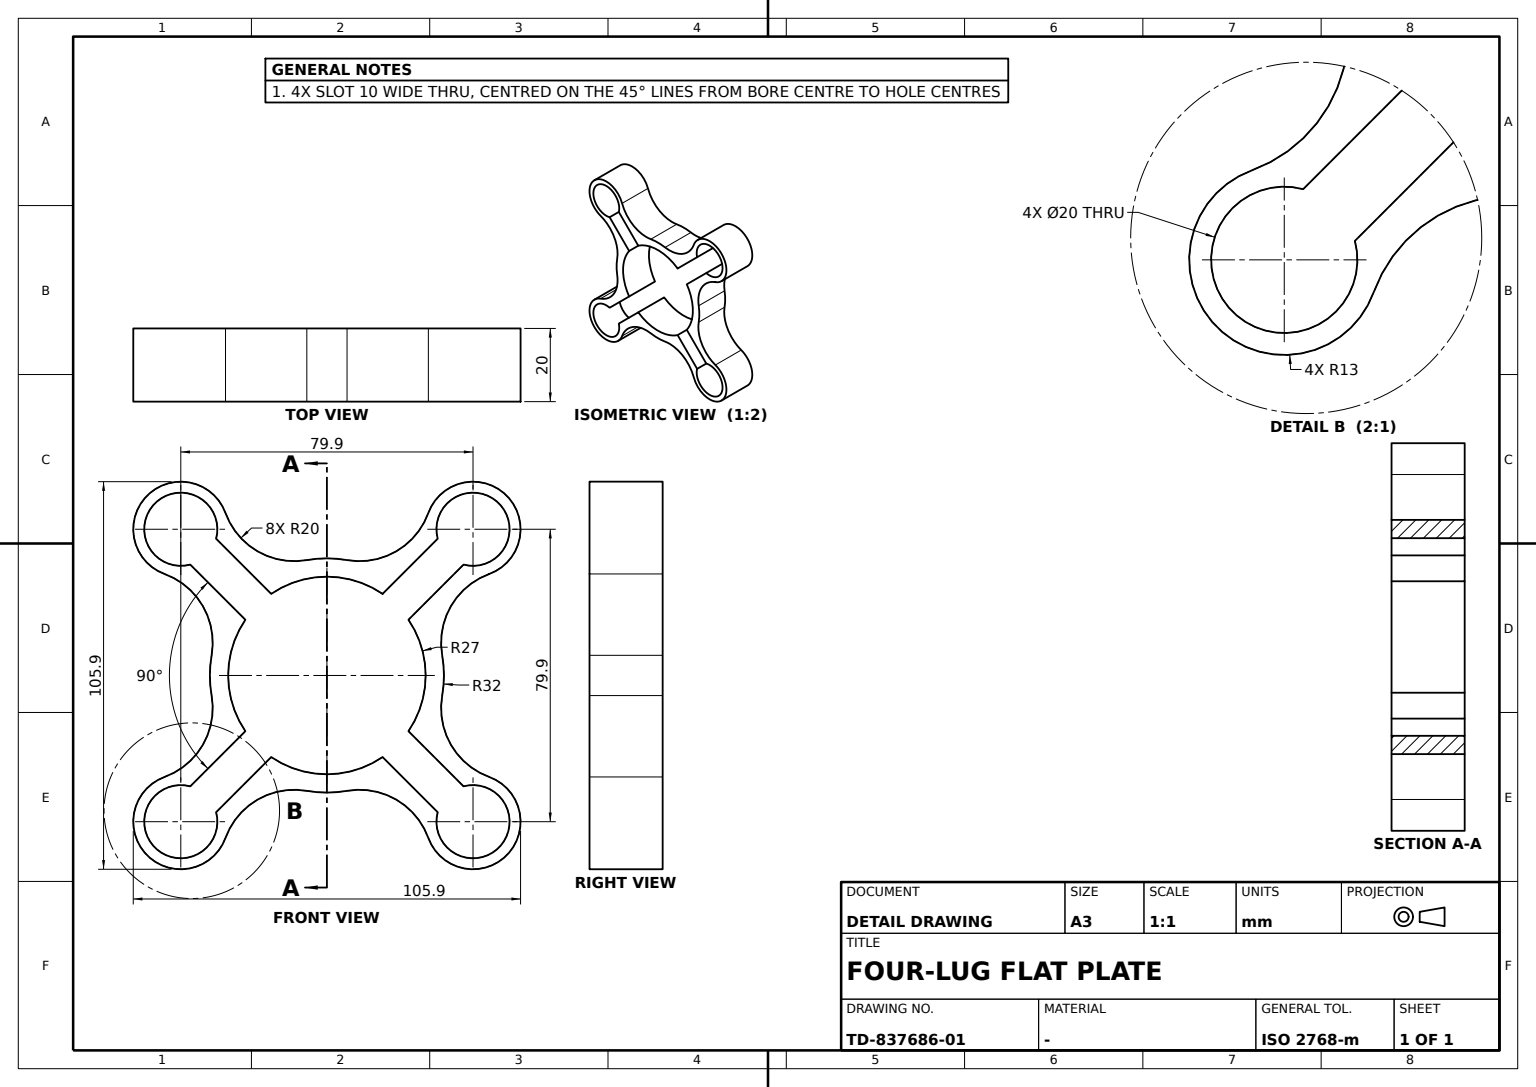
ISO-10303-21;
HEADER;
FILE_DESCRIPTION((''),'2;1');
FILE_NAME('','',(''),(''),'','','');
FILE_SCHEMA(('AUTOMOTIVE_DESIGN'));
ENDSEC;
DATA;
#1=APPLICATION_CONTEXT('');
#2=PRODUCT_CONTEXT('',#1,'mechanical');
#3=PRODUCT('','','',(#2));
#4=PRODUCT_DEFINITION_FORMATION('','',#3);
#5=PRODUCT_DEFINITION_CONTEXT('',#1,'design');
#6=PRODUCT_DEFINITION('','',#4,#5);
#7=PRODUCT_DEFINITION_SHAPE('','',#6);
#8=(LENGTH_UNIT()NAMED_UNIT(*)SI_UNIT(.MILLI.,.METRE.));
#9=(NAMED_UNIT(*)PLANE_ANGLE_UNIT()SI_UNIT($,.RADIAN.));
#10=(NAMED_UNIT(*)SI_UNIT($,.STERADIAN.)SOLID_ANGLE_UNIT());
#11=UNCERTAINTY_MEASURE_WITH_UNIT(LENGTH_MEASURE(0.005),#8,'distance_accuracy_value','');
#12=(GEOMETRIC_REPRESENTATION_CONTEXT(3)GLOBAL_UNCERTAINTY_ASSIGNED_CONTEXT((#11))GLOBAL_UNIT_ASSIGNED_CONTEXT((#8,#9,#10))REPRESENTATION_CONTEXT('',''));
#13=CARTESIAN_POINT('',(-10.,30.292275,37.363343));
#14=VERTEX_POINT('',#13);
#15=CARTESIAN_POINT('',(10.,30.292275,37.363343));
#16=VERTEX_POINT('',#15);
#17=DIRECTION('',(1.,0.,0.));
#18=VECTOR('',#17,1000.);
#19=LINE('',#13,#18);
#20=EDGE_CURVE('',#14,#16,#19,.T.);
#21=ORIENTED_EDGE('',*,*,#20,.F.);
#22=CARTESIAN_POINT('',(-10.,37.363343,30.292275));
#23=VERTEX_POINT('',#22);
#24=CARTESIAN_POINT('',(-10.,39.951533,39.951533));
#25=DIRECTION('',(0.,0.,-1.));
#26=AXIS2_PLACEMENT_3D('',#24,#17,#25);
#27=CIRCLE('',#26,10.);
#28=EDGE_CURVE('',#23,#14,#27,.T.);
#29=ORIENTED_EDGE('',*,*,#28,.F.);
#30=CARTESIAN_POINT('',(10.,37.363343,30.292275));
#31=VERTEX_POINT('',#30);
#32=LINE('',#22,#18);
#33=EDGE_CURVE('',#23,#31,#32,.T.);
#34=ORIENTED_EDGE('',*,*,#33,.T.);
#35=CARTESIAN_POINT('',(10.,39.951533,39.951533));
#36=AXIS2_PLACEMENT_3D('',#35,#17,#25);
#37=CIRCLE('',#36,10.);
#38=EDGE_CURVE('',#31,#16,#37,.T.);
#39=ORIENTED_EDGE('',*,*,#38,.T.);
#40=EDGE_LOOP('',(#21,#29,#34,#39));
#41=FACE_BOUND('',#40,.T.);
#42=CARTESIAN_POINT('',(0.,39.951533,39.951533));
#43=DIRECTION('',(0.,1.,0.));
#44=AXIS2_PLACEMENT_3D('',#42,#17,#43);
#45=CYLINDRICAL_SURFACE('',#44,10.);
#46=ADVANCED_FACE('',(#41),#45,.F.);
#47=CARTESIAN_POINT('',(-10.,-44.393072,-27.733811));
#48=VERTEX_POINT('',#47);
#49=CARTESIAN_POINT('',(10.,-44.393072,-27.733811));
#50=VERTEX_POINT('',#49);
#51=CARTESIAN_POINT('',(0.,-44.393072,-27.733811));
#52=LINE('',#51,#18);
#53=EDGE_CURVE('',#48,#50,#52,.T.);
#54=ORIENTED_EDGE('',*,*,#53,.T.);
#55=CARTESIAN_POINT('',(10.,-31.52382,-5.499886));
#56=VERTEX_POINT('',#55);
#57=CARTESIAN_POINT('',(10.,-51.226208,-8.937315));
#58=AXIS2_PLACEMENT_3D('',#57,#17,#25);
#59=CIRCLE('',#58,20.);
#60=EDGE_CURVE('',#50,#56,#59,.T.);
#61=ORIENTED_EDGE('',*,*,#60,.T.);
#62=CARTESIAN_POINT('',(-10.,-31.52382,-5.499886));
#63=VERTEX_POINT('',#62);
#64=CARTESIAN_POINT('',(0.,-31.52382,-5.499886));
#65=LINE('',#64,#18);
#66=EDGE_CURVE('',#63,#56,#65,.T.);
#67=ORIENTED_EDGE('',*,*,#66,.F.);
#68=CARTESIAN_POINT('',(-10.,-51.226208,-8.937315));
#69=AXIS2_PLACEMENT_3D('',#68,#17,#25);
#70=CIRCLE('',#69,20.);
#71=EDGE_CURVE('',#48,#63,#70,.T.);
#72=ORIENTED_EDGE('',*,*,#71,.F.);
#73=EDGE_LOOP('',(#54,#61,#67,#72));
#74=FACE_BOUND('',#73,.T.);
#75=CARTESIAN_POINT('',(0.,-51.226208,-8.937315));
#76=AXIS2_PLACEMENT_3D('',#75,#17,#43);
#77=CYLINDRICAL_SURFACE('',#76,20.);
#78=ADVANCED_FACE('',(#74),#77,.F.);
#79=CARTESIAN_POINT('',(-10.,-37.363343,-30.292275));
#80=VERTEX_POINT('',#79);
#81=CARTESIAN_POINT('',(10.,-37.363343,-30.292275));
#82=VERTEX_POINT('',#81);
#83=LINE('',#79,#18);
#84=EDGE_CURVE('',#80,#82,#83,.T.);
#85=ORIENTED_EDGE('',*,*,#84,.F.);
#86=CARTESIAN_POINT('',(-10.,-22.297197,-15.226129));
#87=VERTEX_POINT('',#86);
#88=CARTESIAN_POINT('',(-10.,-3.535534,3.535534));
#89=DIRECTION('',(0.,-0.707106781,-0.707106781));
#90=VECTOR('',#89,1000.);
#91=LINE('',#88,#90);
#92=EDGE_CURVE('',#87,#80,#91,.T.);
#93=ORIENTED_EDGE('',*,*,#92,.F.);
#94=CARTESIAN_POINT('',(10.,-22.297197,-15.226129));
#95=VERTEX_POINT('',#94);
#96=LINE('',#86,#18);
#97=EDGE_CURVE('',#87,#95,#96,.T.);
#98=ORIENTED_EDGE('',*,*,#97,.T.);
#99=CARTESIAN_POINT('',(10.,-3.535534,3.535534));
#100=LINE('',#99,#90);
#101=EDGE_CURVE('',#95,#82,#100,.T.);
#102=ORIENTED_EDGE('',*,*,#101,.T.);
#103=EDGE_LOOP('',(#85,#93,#98,#102));
#104=FACE_BOUND('',#103,.T.);
#105=CARTESIAN_POINT('',(0.,-22.297197,-15.226129));
#106=DIRECTION('',(0.,-0.707106781,0.707106781));
#107=AXIS2_PLACEMENT_3D('',#105,#106,#89);
#108=PLANE('',#107);
#109=ADVANCED_FACE('',(#104),#108,.F.);
#110=CARTESIAN_POINT('',(10.,-15.226129,-22.297197));
#111=VERTEX_POINT('',#110);
#112=CARTESIAN_POINT('',(10.,15.226129,-22.297197));
#113=VERTEX_POINT('',#112);
#114=CARTESIAN_POINT('',(10.,0.,0.));
#115=AXIS2_PLACEMENT_3D('',#114,#17,#25);
#116=CIRCLE('',#115,27.);
#117=EDGE_CURVE('',#111,#113,#116,.T.);
#118=ORIENTED_EDGE('',*,*,#117,.T.);
#119=CARTESIAN_POINT('',(-10.,15.226129,-22.297197));
#120=VERTEX_POINT('',#119);
#121=LINE('',#119,#18);
#122=EDGE_CURVE('',#120,#113,#121,.T.);
#123=ORIENTED_EDGE('',*,*,#122,.F.);
#124=CARTESIAN_POINT('',(-10.,-15.226129,-22.297197));
#125=VERTEX_POINT('',#124);
#126=CARTESIAN_POINT('',(-10.,0.,0.));
#127=AXIS2_PLACEMENT_3D('',#126,#17,#25);
#128=CIRCLE('',#127,27.);
#129=EDGE_CURVE('',#125,#120,#128,.T.);
#130=ORIENTED_EDGE('',*,*,#129,.F.);
#131=LINE('',#124,#18);
#132=EDGE_CURVE('',#125,#111,#131,.T.);
#133=ORIENTED_EDGE('',*,*,#132,.T.);
#134=EDGE_LOOP('',(#118,#123,#130,#133));
#135=FACE_BOUND('',#134,.T.);
#136=CARTESIAN_POINT('',(0.,0.,0.));
#137=AXIS2_PLACEMENT_3D('',#136,#17,#43);
#138=CYLINDRICAL_SURFACE('',#137,27.);
#139=ADVANCED_FACE('',(#135),#138,.F.);
#140=CARTESIAN_POINT('',(-10.,44.393072,-27.733811));
#141=VERTEX_POINT('',#140);
#142=CARTESIAN_POINT('',(10.,44.393072,-27.733811));
#143=VERTEX_POINT('',#142);
#144=CARTESIAN_POINT('',(0.,44.393072,-27.733811));
#145=LINE('',#144,#18);
#146=EDGE_CURVE('',#141,#143,#145,.T.);
#147=ORIENTED_EDGE('',*,*,#146,.F.);
#148=CARTESIAN_POINT('',(-10.,31.52382,-5.499886));
#149=VERTEX_POINT('',#148);
#150=CARTESIAN_POINT('',(-10.,51.226208,-8.937315));
#151=AXIS2_PLACEMENT_3D('',#150,#17,#25);
#152=CIRCLE('',#151,20.);
#153=EDGE_CURVE('',#149,#141,#152,.T.);
#154=ORIENTED_EDGE('',*,*,#153,.F.);
#155=CARTESIAN_POINT('',(10.,31.52382,-5.499886));
#156=VERTEX_POINT('',#155);
#157=CARTESIAN_POINT('',(0.,31.52382,-5.499886));
#158=LINE('',#157,#18);
#159=EDGE_CURVE('',#149,#156,#158,.T.);
#160=ORIENTED_EDGE('',*,*,#159,.T.);
#161=CARTESIAN_POINT('',(10.,51.226208,-8.937315));
#162=AXIS2_PLACEMENT_3D('',#161,#17,#25);
#163=CIRCLE('',#162,20.);
#164=EDGE_CURVE('',#156,#143,#163,.T.);
#165=ORIENTED_EDGE('',*,*,#164,.T.);
#166=EDGE_LOOP('',(#147,#154,#160,#165));
#167=FACE_BOUND('',#166,.T.);
#168=CARTESIAN_POINT('',(0.,51.226208,-8.937315));
#169=AXIS2_PLACEMENT_3D('',#168,#17,#43);
#170=CYLINDRICAL_SURFACE('',#169,20.);
#171=ADVANCED_FACE('',(#167),#170,.F.);
#172=CARTESIAN_POINT('',(-10.,30.292275,-37.363343));
#173=VERTEX_POINT('',#172);
#174=CARTESIAN_POINT('',(-10.,37.363343,-30.292275));
#175=VERTEX_POINT('',#174);
#176=CARTESIAN_POINT('',(-10.,39.951533,-39.951533));
#177=AXIS2_PLACEMENT_3D('',#176,#17,#25);
#178=CIRCLE('',#177,10.);
#179=EDGE_CURVE('',#173,#175,#178,.T.);
#180=ORIENTED_EDGE('',*,*,#179,.F.);
#181=CARTESIAN_POINT('',(10.,30.292275,-37.363343));
#182=VERTEX_POINT('',#181);
#183=LINE('',#172,#18);
#184=EDGE_CURVE('',#173,#182,#183,.T.);
#185=ORIENTED_EDGE('',*,*,#184,.T.);
#186=CARTESIAN_POINT('',(10.,37.363343,-30.292275));
#187=VERTEX_POINT('',#186);
#188=CARTESIAN_POINT('',(10.,39.951533,-39.951533));
#189=AXIS2_PLACEMENT_3D('',#188,#17,#25);
#190=CIRCLE('',#189,10.);
#191=EDGE_CURVE('',#182,#187,#190,.T.);
#192=ORIENTED_EDGE('',*,*,#191,.T.);
#193=LINE('',#174,#18);
#194=EDGE_CURVE('',#175,#187,#193,.T.);
#195=ORIENTED_EDGE('',*,*,#194,.F.);
#196=EDGE_LOOP('',(#180,#185,#192,#195));
#197=FACE_BOUND('',#196,.T.);
#198=CARTESIAN_POINT('',(0.,39.951533,-39.951533));
#199=AXIS2_PLACEMENT_3D('',#198,#17,#43);
#200=CYLINDRICAL_SURFACE('',#199,10.);
#201=ADVANCED_FACE('',(#197),#200,.F.);
#202=CARTESIAN_POINT('',(-10.,-37.363343,30.292275));
#203=VERTEX_POINT('',#202);
#204=CARTESIAN_POINT('',(10.,-37.363343,30.292275));
#205=VERTEX_POINT('',#204);
#206=LINE('',#202,#18);
#207=EDGE_CURVE('',#203,#205,#206,.T.);
#208=ORIENTED_EDGE('',*,*,#207,.F.);
#209=CARTESIAN_POINT('',(-10.,-30.292275,37.363343));
#210=VERTEX_POINT('',#209);
#211=CARTESIAN_POINT('',(-10.,-39.951533,39.951533));
#212=AXIS2_PLACEMENT_3D('',#211,#17,#25);
#213=CIRCLE('',#212,10.);
#214=EDGE_CURVE('',#210,#203,#213,.T.);
#215=ORIENTED_EDGE('',*,*,#214,.F.);
#216=CARTESIAN_POINT('',(10.,-30.292275,37.363343));
#217=VERTEX_POINT('',#216);
#218=LINE('',#209,#18);
#219=EDGE_CURVE('',#210,#217,#218,.T.);
#220=ORIENTED_EDGE('',*,*,#219,.T.);
#221=CARTESIAN_POINT('',(10.,-39.951533,39.951533));
#222=AXIS2_PLACEMENT_3D('',#221,#17,#25);
#223=CIRCLE('',#222,10.);
#224=EDGE_CURVE('',#217,#205,#223,.T.);
#225=ORIENTED_EDGE('',*,*,#224,.T.);
#226=EDGE_LOOP('',(#208,#215,#220,#225));
#227=FACE_BOUND('',#226,.T.);
#228=CARTESIAN_POINT('',(0.,-39.951533,39.951533));
#229=AXIS2_PLACEMENT_3D('',#228,#17,#43);
#230=CYLINDRICAL_SURFACE('',#229,10.);
#231=ADVANCED_FACE('',(#227),#230,.F.);
#232=CARTESIAN_POINT('',(10.,31.52382,5.499886));
#233=VERTEX_POINT('',#232);
#234=CIRCLE('',#115,32.);
#235=EDGE_CURVE('',#156,#233,#234,.T.);
#236=ORIENTED_EDGE('',*,*,#235,.F.);
#237=ORIENTED_EDGE('',*,*,#159,.F.);
#238=CARTESIAN_POINT('',(-10.,31.52382,5.499886));
#239=VERTEX_POINT('',#238);
#240=CIRCLE('',#127,32.);
#241=EDGE_CURVE('',#149,#239,#240,.T.);
#242=ORIENTED_EDGE('',*,*,#241,.T.);
#243=CARTESIAN_POINT('',(0.,31.52382,5.499886));
#244=LINE('',#243,#18);
#245=EDGE_CURVE('',#239,#233,#244,.T.);
#246=ORIENTED_EDGE('',*,*,#245,.T.);
#247=EDGE_LOOP('',(#236,#237,#242,#246));
#248=FACE_BOUND('',#247,.T.);
#249=CYLINDRICAL_SURFACE('',#137,32.);
#250=ADVANCED_FACE('',(#248),#249,.T.);
#251=CARTESIAN_POINT('',(-10.,-15.226129,22.297197));
#252=VERTEX_POINT('',#251);
#253=CARTESIAN_POINT('',(10.,-15.226129,22.297197));
#254=VERTEX_POINT('',#253);
#255=LINE('',#251,#18);
#256=EDGE_CURVE('',#252,#254,#255,.T.);
#257=ORIENTED_EDGE('',*,*,#256,.T.);
#258=CARTESIAN_POINT('',(10.,3.535534,3.535534));
#259=VECTOR('',#106,1000.);
#260=LINE('',#258,#259);
#261=EDGE_CURVE('',#254,#217,#260,.T.);
#262=ORIENTED_EDGE('',*,*,#261,.T.);
#263=ORIENTED_EDGE('',*,*,#219,.F.);
#264=CARTESIAN_POINT('',(-10.,3.535534,3.535534));
#265=LINE('',#264,#259);
#266=EDGE_CURVE('',#252,#210,#265,.T.);
#267=ORIENTED_EDGE('',*,*,#266,.F.);
#268=EDGE_LOOP('',(#257,#262,#263,#267));
#269=FACE_BOUND('',#268,.T.);
#270=CARTESIAN_POINT('',(0.,-15.226129,22.297197));
#271=DIRECTION('',(0.,0.707106781,0.707106781));
#272=AXIS2_PLACEMENT_3D('',#270,#271,#106);
#273=PLANE('',#272);
#274=ADVANCED_FACE('',(#269),#273,.F.);
#275=CARTESIAN_POINT('',(10.,-5.499886,-31.52382));
#276=VERTEX_POINT('',#275);
#277=CARTESIAN_POINT('',(10.,5.499886,-31.52382));
#278=VERTEX_POINT('',#277);
#279=EDGE_CURVE('',#276,#278,#234,.T.);
#280=ORIENTED_EDGE('',*,*,#279,.F.);
#281=CARTESIAN_POINT('',(-10.,-5.499886,-31.52382));
#282=VERTEX_POINT('',#281);
#283=CARTESIAN_POINT('',(0.,-5.499886,-31.52382));
#284=LINE('',#283,#18);
#285=EDGE_CURVE('',#282,#276,#284,.T.);
#286=ORIENTED_EDGE('',*,*,#285,.F.);
#287=CARTESIAN_POINT('',(-10.,5.499886,-31.52382));
#288=VERTEX_POINT('',#287);
#289=EDGE_CURVE('',#282,#288,#240,.T.);
#290=ORIENTED_EDGE('',*,*,#289,.T.);
#291=CARTESIAN_POINT('',(0.,5.499886,-31.52382));
#292=LINE('',#291,#18);
#293=EDGE_CURVE('',#288,#278,#292,.T.);
#294=ORIENTED_EDGE('',*,*,#293,.T.);
#295=EDGE_LOOP('',(#280,#286,#290,#294));
#296=FACE_BOUND('',#295,.T.);
#297=ADVANCED_FACE('',(#296),#249,.T.);
#298=CARTESIAN_POINT('',(-10.,-27.733811,44.393072));
#299=VERTEX_POINT('',#298);
#300=CARTESIAN_POINT('',(10.,-27.733811,44.393072));
#301=VERTEX_POINT('',#300);
#302=CARTESIAN_POINT('',(0.,-27.733811,44.393072));
#303=LINE('',#302,#18);
#304=EDGE_CURVE('',#299,#301,#303,.T.);
#305=ORIENTED_EDGE('',*,*,#304,.T.);
#306=CARTESIAN_POINT('',(10.,-5.499886,31.52382));
#307=VERTEX_POINT('',#306);
#308=CARTESIAN_POINT('',(10.,-8.937315,51.226208));
#309=AXIS2_PLACEMENT_3D('',#308,#17,#25);
#310=CIRCLE('',#309,20.);
#311=EDGE_CURVE('',#301,#307,#310,.T.);
#312=ORIENTED_EDGE('',*,*,#311,.T.);
#313=CARTESIAN_POINT('',(-10.,-5.499886,31.52382));
#314=VERTEX_POINT('',#313);
#315=CARTESIAN_POINT('',(0.,-5.499886,31.52382));
#316=LINE('',#315,#18);
#317=EDGE_CURVE('',#314,#307,#316,.T.);
#318=ORIENTED_EDGE('',*,*,#317,.F.);
#319=CARTESIAN_POINT('',(-10.,-8.937315,51.226208));
#320=AXIS2_PLACEMENT_3D('',#319,#17,#25);
#321=CIRCLE('',#320,20.);
#322=EDGE_CURVE('',#299,#314,#321,.T.);
#323=ORIENTED_EDGE('',*,*,#322,.F.);
#324=EDGE_LOOP('',(#305,#312,#318,#323));
#325=FACE_BOUND('',#324,.T.);
#326=CARTESIAN_POINT('',(0.,-8.937315,51.226208));
#327=AXIS2_PLACEMENT_3D('',#326,#17,#43);
#328=CYLINDRICAL_SURFACE('',#327,20.);
#329=ADVANCED_FACE('',(#325),#328,.F.);
#330=ORIENTED_EDGE('',*,*,#146,.T.);
#331=CARTESIAN_POINT('',(10.,27.733811,-44.393072));
#332=VERTEX_POINT('',#331);
#333=CIRCLE('',#189,13.);
#334=EDGE_CURVE('',#332,#143,#333,.T.);
#335=ORIENTED_EDGE('',*,*,#334,.F.);
#336=CARTESIAN_POINT('',(-10.,27.733811,-44.393072));
#337=VERTEX_POINT('',#336);
#338=CARTESIAN_POINT('',(0.,27.733811,-44.393072));
#339=LINE('',#338,#18);
#340=EDGE_CURVE('',#337,#332,#339,.T.);
#341=ORIENTED_EDGE('',*,*,#340,.F.);
#342=CIRCLE('',#177,13.);
#343=EDGE_CURVE('',#337,#141,#342,.T.);
#344=ORIENTED_EDGE('',*,*,#343,.T.);
#345=EDGE_LOOP('',(#330,#335,#341,#344));
#346=FACE_BOUND('',#345,.T.);
#347=CYLINDRICAL_SURFACE('',#199,13.);
#348=ADVANCED_FACE('',(#346),#347,.T.);
#349=CARTESIAN_POINT('',(-10.,-22.297197,15.226129));
#350=DIRECTION('',(0.,0.707106781,-0.707106781));
#351=VECTOR('',#350,1000.);
#352=LINE('',#349,#351);
#353=EDGE_CURVE('',#120,#173,#352,.T.);
#354=ORIENTED_EDGE('',*,*,#353,.F.);
#355=ORIENTED_EDGE('',*,*,#122,.T.);
#356=CARTESIAN_POINT('',(10.,-22.297197,15.226129));
#357=LINE('',#356,#351);
#358=EDGE_CURVE('',#113,#182,#357,.T.);
#359=ORIENTED_EDGE('',*,*,#358,.T.);
#360=ORIENTED_EDGE('',*,*,#184,.F.);
#361=EDGE_LOOP('',(#354,#355,#359,#360));
#362=FACE_BOUND('',#361,.T.);
#363=CARTESIAN_POINT('',(0.,-22.297197,15.226129));
#364=AXIS2_PLACEMENT_3D('',#363,#271,#106);
#365=PLANE('',#364);
#366=ADVANCED_FACE('',(#362),#365,.T.);
#367=ORIENTED_EDGE('',*,*,#38,.F.);
#368=CARTESIAN_POINT('',(10.,22.297197,15.226129));
#369=VERTEX_POINT('',#368);
#370=VECTOR('',#271,1000.);
#371=LINE('',#110,#370);
#372=EDGE_CURVE('',#369,#31,#371,.T.);
#373=ORIENTED_EDGE('',*,*,#372,.F.);
#374=CARTESIAN_POINT('',(10.,22.297197,-15.226129));
#375=VERTEX_POINT('',#374);
#376=EDGE_CURVE('',#375,#369,#116,.T.);
#377=ORIENTED_EDGE('',*,*,#376,.F.);
#378=LINE('',#253,#351);
#379=EDGE_CURVE('',#375,#187,#378,.T.);
#380=ORIENTED_EDGE('',*,*,#379,.T.);
#381=ORIENTED_EDGE('',*,*,#191,.F.);
#382=ORIENTED_EDGE('',*,*,#358,.F.);
#383=ORIENTED_EDGE('',*,*,#117,.F.);
#384=CARTESIAN_POINT('',(10.,-30.292275,-37.363343));
#385=VERTEX_POINT('',#384);
#386=CARTESIAN_POINT('',(10.,3.535534,-3.535534));
#387=LINE('',#386,#90);
#388=EDGE_CURVE('',#111,#385,#387,.T.);
#389=ORIENTED_EDGE('',*,*,#388,.T.);
#390=CARTESIAN_POINT('',(10.,-39.951533,-39.951533));
#391=AXIS2_PLACEMENT_3D('',#390,#17,#25);
#392=CIRCLE('',#391,10.);
#393=EDGE_CURVE('',#82,#385,#392,.T.);
#394=ORIENTED_EDGE('',*,*,#393,.F.);
#395=ORIENTED_EDGE('',*,*,#101,.F.);
#396=VERTEX_POINT('',#356);
#397=EDGE_CURVE('',#396,#95,#116,.T.);
#398=ORIENTED_EDGE('',*,*,#397,.F.);
#399=CARTESIAN_POINT('',(10.,-3.535534,-3.535534));
#400=LINE('',#399,#259);
#401=EDGE_CURVE('',#396,#205,#400,.T.);
#402=ORIENTED_EDGE('',*,*,#401,.T.);
#403=ORIENTED_EDGE('',*,*,#224,.F.);
#404=ORIENTED_EDGE('',*,*,#261,.F.);
#405=CARTESIAN_POINT('',(10.,15.226129,22.297197));
#406=VERTEX_POINT('',#405);
#407=EDGE_CURVE('',#406,#254,#116,.T.);
#408=ORIENTED_EDGE('',*,*,#407,.F.);
#409=LINE('',#94,#370);
#410=EDGE_CURVE('',#406,#16,#409,.T.);
#411=ORIENTED_EDGE('',*,*,#410,.T.);
#412=EDGE_LOOP('',(#367,#373,#377,#380,#381,#382,#383,#389,#394,#395,#398,#402,#403,#404,#408,#411));
#413=FACE_BOUND('',#412,.T.);
#414=ORIENTED_EDGE('',*,*,#279,.T.);
#415=CARTESIAN_POINT('',(10.,8.937315,-51.226208));
#416=AXIS2_PLACEMENT_3D('',#415,#17,#25);
#417=CIRCLE('',#416,20.);
#418=EDGE_CURVE('',#332,#278,#417,.T.);
#419=ORIENTED_EDGE('',*,*,#418,.F.);
#420=ORIENTED_EDGE('',*,*,#334,.T.);
#421=ORIENTED_EDGE('',*,*,#164,.F.);
#422=ORIENTED_EDGE('',*,*,#235,.T.);
#423=CARTESIAN_POINT('',(10.,44.393072,27.733811));
#424=VERTEX_POINT('',#423);
#425=CARTESIAN_POINT('',(10.,51.226208,8.937315));
#426=AXIS2_PLACEMENT_3D('',#425,#17,#25);
#427=CIRCLE('',#426,20.);
#428=EDGE_CURVE('',#424,#233,#427,.T.);
#429=ORIENTED_EDGE('',*,*,#428,.F.);
#430=CARTESIAN_POINT('',(10.,27.733811,44.393072));
#431=VERTEX_POINT('',#430);
#432=CIRCLE('',#36,13.);
#433=EDGE_CURVE('',#424,#431,#432,.T.);
#434=ORIENTED_EDGE('',*,*,#433,.T.);
#435=CARTESIAN_POINT('',(10.,5.499886,31.52382));
#436=VERTEX_POINT('',#435);
#437=CARTESIAN_POINT('',(10.,8.937315,51.226208));
#438=AXIS2_PLACEMENT_3D('',#437,#17,#25);
#439=CIRCLE('',#438,20.);
#440=EDGE_CURVE('',#436,#431,#439,.T.);
#441=ORIENTED_EDGE('',*,*,#440,.F.);
#442=EDGE_CURVE('',#436,#307,#234,.T.);
#443=ORIENTED_EDGE('',*,*,#442,.T.);
#444=ORIENTED_EDGE('',*,*,#311,.F.);
#445=CARTESIAN_POINT('',(10.,-44.393072,27.733811));
#446=VERTEX_POINT('',#445);
#447=CIRCLE('',#222,13.);
#448=EDGE_CURVE('',#301,#446,#447,.T.);
#449=ORIENTED_EDGE('',*,*,#448,.T.);
#450=CARTESIAN_POINT('',(10.,-31.52382,5.499886));
#451=VERTEX_POINT('',#450);
#452=CARTESIAN_POINT('',(10.,-51.226208,8.937315));
#453=AXIS2_PLACEMENT_3D('',#452,#17,#25);
#454=CIRCLE('',#453,20.);
#455=EDGE_CURVE('',#451,#446,#454,.T.);
#456=ORIENTED_EDGE('',*,*,#455,.F.);
#457=EDGE_CURVE('',#451,#56,#234,.T.);
#458=ORIENTED_EDGE('',*,*,#457,.T.);
#459=ORIENTED_EDGE('',*,*,#60,.F.);
#460=CARTESIAN_POINT('',(10.,-27.733811,-44.393072));
#461=VERTEX_POINT('',#460);
#462=CIRCLE('',#391,13.);
#463=EDGE_CURVE('',#50,#461,#462,.T.);
#464=ORIENTED_EDGE('',*,*,#463,.T.);
#465=CARTESIAN_POINT('',(10.,-8.937315,-51.226208));
#466=AXIS2_PLACEMENT_3D('',#465,#17,#25);
#467=CIRCLE('',#466,20.);
#468=EDGE_CURVE('',#276,#461,#467,.T.);
#469=ORIENTED_EDGE('',*,*,#468,.F.);
#470=EDGE_LOOP('',(#414,#419,#420,#421,#422,#429,#434,#441,#443,#444,#449,#456,#458,#459,#464,#469));
#471=FACE_BOUND('',#470,.T.);
#472=AXIS2_PLACEMENT_3D('',#114,#17,#43);
#473=PLANE('',#472);
#474=ADVANCED_FACE('',(#413,#471),#473,.T.);
#475=VERTEX_POINT('',#349);
#476=LINE('',#349,#18);
#477=EDGE_CURVE('',#475,#396,#476,.T.);
#478=ORIENTED_EDGE('',*,*,#477,.F.);
#479=CARTESIAN_POINT('',(-10.,-3.535534,-3.535534));
#480=LINE('',#479,#259);
#481=EDGE_CURVE('',#475,#203,#480,.T.);
#482=ORIENTED_EDGE('',*,*,#481,.T.);
#483=ORIENTED_EDGE('',*,*,#207,.T.);
#484=ORIENTED_EDGE('',*,*,#401,.F.);
#485=EDGE_LOOP('',(#478,#482,#483,#484));
#486=FACE_BOUND('',#485,.T.);
#487=ADVANCED_FACE('',(#486),#365,.T.);
#488=CARTESIAN_POINT('',(-10.,8.937315,-51.226208));
#489=AXIS2_PLACEMENT_3D('',#488,#17,#25);
#490=CIRCLE('',#489,20.);
#491=EDGE_CURVE('',#337,#288,#490,.T.);
#492=ORIENTED_EDGE('',*,*,#491,.F.);
#493=ORIENTED_EDGE('',*,*,#340,.T.);
#494=ORIENTED_EDGE('',*,*,#418,.T.);
#495=ORIENTED_EDGE('',*,*,#293,.F.);
#496=EDGE_LOOP('',(#492,#493,#494,#495));
#497=FACE_BOUND('',#496,.T.);
#498=CARTESIAN_POINT('',(0.,8.937315,-51.226208));
#499=AXIS2_PLACEMENT_3D('',#498,#17,#43);
#500=CYLINDRICAL_SURFACE('',#499,20.);
#501=ADVANCED_FACE('',(#497),#500,.F.);
#502=CARTESIAN_POINT('',(-10.,15.226129,22.297197));
#503=VERTEX_POINT('',#502);
#504=LINE('',#502,#18);
#505=EDGE_CURVE('',#503,#406,#504,.T.);
#506=ORIENTED_EDGE('',*,*,#505,.F.);
#507=LINE('',#86,#370);
#508=EDGE_CURVE('',#503,#14,#507,.T.);
#509=ORIENTED_EDGE('',*,*,#508,.T.);
#510=ORIENTED_EDGE('',*,*,#20,.T.);
#511=ORIENTED_EDGE('',*,*,#410,.F.);
#512=EDGE_LOOP('',(#506,#509,#510,#511));
#513=FACE_BOUND('',#512,.T.);
#514=ADVANCED_FACE('',(#513),#108,.F.);
#515=ORIENTED_EDGE('',*,*,#372,.T.);
#516=ORIENTED_EDGE('',*,*,#33,.F.);
#517=CARTESIAN_POINT('',(-10.,22.297197,15.226129));
#518=VERTEX_POINT('',#517);
#519=LINE('',#124,#370);
#520=EDGE_CURVE('',#518,#23,#519,.T.);
#521=ORIENTED_EDGE('',*,*,#520,.F.);
#522=LINE('',#517,#18);
#523=EDGE_CURVE('',#518,#369,#522,.T.);
#524=ORIENTED_EDGE('',*,*,#523,.T.);
#525=EDGE_LOOP('',(#515,#516,#521,#524));
#526=FACE_BOUND('',#525,.T.);
#527=CARTESIAN_POINT('',(0.,-15.226129,-22.297197));
#528=AXIS2_PLACEMENT_3D('',#527,#106,#89);
#529=PLANE('',#528);
#530=ADVANCED_FACE('',(#526),#529,.T.);
#531=CARTESIAN_POINT('',(-10.,22.297197,-15.226129));
#532=VERTEX_POINT('',#531);
#533=LINE('',#531,#18);
#534=EDGE_CURVE('',#532,#375,#533,.T.);
#535=ORIENTED_EDGE('',*,*,#534,.F.);
#536=LINE('',#251,#351);
#537=EDGE_CURVE('',#532,#175,#536,.T.);
#538=ORIENTED_EDGE('',*,*,#537,.T.);
#539=ORIENTED_EDGE('',*,*,#194,.T.);
#540=ORIENTED_EDGE('',*,*,#379,.F.);
#541=EDGE_LOOP('',(#535,#538,#539,#540));
#542=FACE_BOUND('',#541,.T.);
#543=ADVANCED_FACE('',(#542),#273,.F.);
#544=ORIENTED_EDGE('',*,*,#317,.T.);
#545=ORIENTED_EDGE('',*,*,#442,.F.);
#546=CARTESIAN_POINT('',(-10.,5.499886,31.52382));
#547=VERTEX_POINT('',#546);
#548=CARTESIAN_POINT('',(0.,5.499886,31.52382));
#549=LINE('',#548,#18);
#550=EDGE_CURVE('',#547,#436,#549,.T.);
#551=ORIENTED_EDGE('',*,*,#550,.F.);
#552=EDGE_CURVE('',#547,#314,#240,.T.);
#553=ORIENTED_EDGE('',*,*,#552,.T.);
#554=EDGE_LOOP('',(#544,#545,#551,#553));
#555=FACE_BOUND('',#554,.T.);
#556=ADVANCED_FACE('',(#555),#249,.T.);
#557=CARTESIAN_POINT('',(-10.,44.393072,27.733811));
#558=VERTEX_POINT('',#557);
#559=CARTESIAN_POINT('',(-10.,27.733811,44.393072));
#560=VERTEX_POINT('',#559);
#561=CIRCLE('',#26,13.);
#562=EDGE_CURVE('',#558,#560,#561,.T.);
#563=ORIENTED_EDGE('',*,*,#562,.T.);
#564=CARTESIAN_POINT('',(0.,27.733811,44.393072));
#565=LINE('',#564,#18);
#566=EDGE_CURVE('',#560,#431,#565,.T.);
#567=ORIENTED_EDGE('',*,*,#566,.T.);
#568=ORIENTED_EDGE('',*,*,#433,.F.);
#569=CARTESIAN_POINT('',(0.,44.393072,27.733811));
#570=LINE('',#569,#18);
#571=EDGE_CURVE('',#558,#424,#570,.T.);
#572=ORIENTED_EDGE('',*,*,#571,.F.);
#573=EDGE_LOOP('',(#563,#567,#568,#572));
#574=FACE_BOUND('',#573,.T.);
#575=CYLINDRICAL_SURFACE('',#44,13.);
#576=ADVANCED_FACE('',(#574),#575,.T.);
#577=ORIENTED_EDGE('',*,*,#66,.T.);
#578=ORIENTED_EDGE('',*,*,#457,.F.);
#579=CARTESIAN_POINT('',(-10.,-31.52382,5.499886));
#580=VERTEX_POINT('',#579);
#581=CARTESIAN_POINT('',(0.,-31.52382,5.499886));
#582=LINE('',#581,#18);
#583=EDGE_CURVE('',#580,#451,#582,.T.);
#584=ORIENTED_EDGE('',*,*,#583,.F.);
#585=EDGE_CURVE('',#580,#63,#240,.T.);
#586=ORIENTED_EDGE('',*,*,#585,.T.);
#587=EDGE_LOOP('',(#577,#578,#584,#586));
#588=FACE_BOUND('',#587,.T.);
#589=ADVANCED_FACE('',(#588),#249,.T.);
#590=CARTESIAN_POINT('',(-10.,-30.292275,-37.363343));
#591=VERTEX_POINT('',#590);
#592=LINE('',#590,#18);
#593=EDGE_CURVE('',#591,#385,#592,.T.);
#594=ORIENTED_EDGE('',*,*,#593,.F.);
#595=CARTESIAN_POINT('',(-10.,-39.951533,-39.951533));
#596=AXIS2_PLACEMENT_3D('',#595,#17,#25);
#597=CIRCLE('',#596,10.);
#598=EDGE_CURVE('',#80,#591,#597,.T.);
#599=ORIENTED_EDGE('',*,*,#598,.F.);
#600=ORIENTED_EDGE('',*,*,#84,.T.);
#601=ORIENTED_EDGE('',*,*,#393,.T.);
#602=EDGE_LOOP('',(#594,#599,#600,#601));
#603=FACE_BOUND('',#602,.T.);
#604=CARTESIAN_POINT('',(0.,-39.951533,-39.951533));
#605=AXIS2_PLACEMENT_3D('',#604,#17,#43);
#606=CYLINDRICAL_SURFACE('',#605,10.);
#607=ADVANCED_FACE('',(#603),#606,.F.);
#608=CARTESIAN_POINT('',(-10.,-44.393072,27.733811));
#609=VERTEX_POINT('',#608);
#610=CIRCLE('',#212,13.);
#611=EDGE_CURVE('',#299,#609,#610,.T.);
#612=ORIENTED_EDGE('',*,*,#611,.T.);
#613=CARTESIAN_POINT('',(0.,-44.393072,27.733811));
#614=LINE('',#613,#18);
#615=EDGE_CURVE('',#609,#446,#614,.T.);
#616=ORIENTED_EDGE('',*,*,#615,.T.);
#617=ORIENTED_EDGE('',*,*,#448,.F.);
#618=ORIENTED_EDGE('',*,*,#304,.F.);
#619=EDGE_LOOP('',(#612,#616,#617,#618));
#620=FACE_BOUND('',#619,.T.);
#621=CYLINDRICAL_SURFACE('',#229,13.);
#622=ADVANCED_FACE('',(#620),#621,.T.);
#623=CARTESIAN_POINT('',(-10.,8.937315,51.226208));
#624=AXIS2_PLACEMENT_3D('',#623,#17,#25);
#625=CIRCLE('',#624,20.);
#626=EDGE_CURVE('',#547,#560,#625,.T.);
#627=ORIENTED_EDGE('',*,*,#626,.F.);
#628=ORIENTED_EDGE('',*,*,#550,.T.);
#629=ORIENTED_EDGE('',*,*,#440,.T.);
#630=ORIENTED_EDGE('',*,*,#566,.F.);
#631=EDGE_LOOP('',(#627,#628,#629,#630));
#632=FACE_BOUND('',#631,.T.);
#633=CARTESIAN_POINT('',(0.,8.937315,51.226208));
#634=AXIS2_PLACEMENT_3D('',#633,#17,#43);
#635=CYLINDRICAL_SURFACE('',#634,20.);
#636=ADVANCED_FACE('',(#632),#635,.F.);
#637=CARTESIAN_POINT('',(-10.,-27.733811,-44.393072));
#638=VERTEX_POINT('',#637);
#639=CARTESIAN_POINT('',(-10.,-8.937315,-51.226208));
#640=AXIS2_PLACEMENT_3D('',#639,#17,#25);
#641=CIRCLE('',#640,20.);
#642=EDGE_CURVE('',#282,#638,#641,.T.);
#643=ORIENTED_EDGE('',*,*,#642,.F.);
#644=ORIENTED_EDGE('',*,*,#285,.T.);
#645=ORIENTED_EDGE('',*,*,#468,.T.);
#646=CARTESIAN_POINT('',(0.,-27.733811,-44.393072));
#647=LINE('',#646,#18);
#648=EDGE_CURVE('',#638,#461,#647,.T.);
#649=ORIENTED_EDGE('',*,*,#648,.F.);
#650=EDGE_LOOP('',(#643,#644,#645,#649));
#651=FACE_BOUND('',#650,.T.);
#652=CARTESIAN_POINT('',(0.,-8.937315,-51.226208));
#653=AXIS2_PLACEMENT_3D('',#652,#17,#43);
#654=CYLINDRICAL_SURFACE('',#653,20.);
#655=ADVANCED_FACE('',(#651),#654,.F.);
#656=ORIENTED_EDGE('',*,*,#53,.F.);
#657=CIRCLE('',#596,13.);
#658=EDGE_CURVE('',#48,#638,#657,.T.);
#659=ORIENTED_EDGE('',*,*,#658,.T.);
#660=ORIENTED_EDGE('',*,*,#648,.T.);
#661=ORIENTED_EDGE('',*,*,#463,.F.);
#662=EDGE_LOOP('',(#656,#659,#660,#661));
#663=FACE_BOUND('',#662,.T.);
#664=CYLINDRICAL_SURFACE('',#605,13.);
#665=ADVANCED_FACE('',(#663),#664,.T.);
#666=ORIENTED_EDGE('',*,*,#245,.F.);
#667=CARTESIAN_POINT('',(-10.,51.226208,8.937315));
#668=AXIS2_PLACEMENT_3D('',#667,#17,#25);
#669=CIRCLE('',#668,20.);
#670=EDGE_CURVE('',#558,#239,#669,.T.);
#671=ORIENTED_EDGE('',*,*,#670,.F.);
#672=ORIENTED_EDGE('',*,*,#571,.T.);
#673=ORIENTED_EDGE('',*,*,#428,.T.);
#674=EDGE_LOOP('',(#666,#671,#672,#673));
#675=FACE_BOUND('',#674,.T.);
#676=CARTESIAN_POINT('',(0.,51.226208,8.937315));
#677=AXIS2_PLACEMENT_3D('',#676,#17,#43);
#678=CYLINDRICAL_SURFACE('',#677,20.);
#679=ADVANCED_FACE('',(#675),#678,.F.);
#680=ORIENTED_EDGE('',*,*,#615,.F.);
#681=CARTESIAN_POINT('',(-10.,-51.226208,8.937315));
#682=AXIS2_PLACEMENT_3D('',#681,#17,#25);
#683=CIRCLE('',#682,20.);
#684=EDGE_CURVE('',#580,#609,#683,.T.);
#685=ORIENTED_EDGE('',*,*,#684,.F.);
#686=ORIENTED_EDGE('',*,*,#583,.T.);
#687=ORIENTED_EDGE('',*,*,#455,.T.);
#688=EDGE_LOOP('',(#680,#685,#686,#687));
#689=FACE_BOUND('',#688,.T.);
#690=CARTESIAN_POINT('',(0.,-51.226208,8.937315));
#691=AXIS2_PLACEMENT_3D('',#690,#17,#43);
#692=CYLINDRICAL_SURFACE('',#691,20.);
#693=ADVANCED_FACE('',(#689),#692,.F.);
#694=EDGE_CURVE('',#532,#518,#128,.T.);
#695=ORIENTED_EDGE('',*,*,#694,.F.);
#696=ORIENTED_EDGE('',*,*,#534,.T.);
#697=ORIENTED_EDGE('',*,*,#376,.T.);
#698=ORIENTED_EDGE('',*,*,#523,.F.);
#699=EDGE_LOOP('',(#695,#696,#697,#698));
#700=FACE_BOUND('',#699,.T.);
#701=ADVANCED_FACE('',(#700),#138,.F.);
#702=CARTESIAN_POINT('',(-10.,3.535534,-3.535534));
#703=LINE('',#702,#90);
#704=EDGE_CURVE('',#125,#591,#703,.T.);
#705=ORIENTED_EDGE('',*,*,#704,.T.);
#706=ORIENTED_EDGE('',*,*,#593,.T.);
#707=ORIENTED_EDGE('',*,*,#388,.F.);
#708=ORIENTED_EDGE('',*,*,#132,.F.);
#709=EDGE_LOOP('',(#705,#706,#707,#708));
#710=FACE_BOUND('',#709,.T.);
#711=ADVANCED_FACE('',(#710),#529,.T.);
#712=ORIENTED_EDGE('',*,*,#241,.F.);
#713=ORIENTED_EDGE('',*,*,#153,.T.);
#714=ORIENTED_EDGE('',*,*,#343,.F.);
#715=ORIENTED_EDGE('',*,*,#491,.T.);
#716=ORIENTED_EDGE('',*,*,#289,.F.);
#717=ORIENTED_EDGE('',*,*,#642,.T.);
#718=ORIENTED_EDGE('',*,*,#658,.F.);
#719=ORIENTED_EDGE('',*,*,#71,.T.);
#720=ORIENTED_EDGE('',*,*,#585,.F.);
#721=ORIENTED_EDGE('',*,*,#684,.T.);
#722=ORIENTED_EDGE('',*,*,#611,.F.);
#723=ORIENTED_EDGE('',*,*,#322,.T.);
#724=ORIENTED_EDGE('',*,*,#552,.F.);
#725=ORIENTED_EDGE('',*,*,#626,.T.);
#726=ORIENTED_EDGE('',*,*,#562,.F.);
#727=ORIENTED_EDGE('',*,*,#670,.T.);
#728=EDGE_LOOP('',(#712,#713,#714,#715,#716,#717,#718,#719,#720,#721,#722,#723,#724,#725,#726,#727));
#729=FACE_BOUND('',#728,.T.);
#730=ORIENTED_EDGE('',*,*,#129,.T.);
#731=ORIENTED_EDGE('',*,*,#353,.T.);
#732=ORIENTED_EDGE('',*,*,#179,.T.);
#733=ORIENTED_EDGE('',*,*,#537,.F.);
#734=ORIENTED_EDGE('',*,*,#694,.T.);
#735=ORIENTED_EDGE('',*,*,#520,.T.);
#736=ORIENTED_EDGE('',*,*,#28,.T.);
#737=ORIENTED_EDGE('',*,*,#508,.F.);
#738=EDGE_CURVE('',#503,#252,#128,.T.);
#739=ORIENTED_EDGE('',*,*,#738,.T.);
#740=ORIENTED_EDGE('',*,*,#266,.T.);
#741=ORIENTED_EDGE('',*,*,#214,.T.);
#742=ORIENTED_EDGE('',*,*,#481,.F.);
#743=EDGE_CURVE('',#475,#87,#128,.T.);
#744=ORIENTED_EDGE('',*,*,#743,.T.);
#745=ORIENTED_EDGE('',*,*,#92,.T.);
#746=ORIENTED_EDGE('',*,*,#598,.T.);
#747=ORIENTED_EDGE('',*,*,#704,.F.);
#748=EDGE_LOOP('',(#730,#731,#732,#733,#734,#735,#736,#737,#739,#740,#741,#742,#744,#745,#746,#747));
#749=FACE_BOUND('',#748,.T.);
#750=AXIS2_PLACEMENT_3D('',#126,#17,#43);
#751=PLANE('',#750);
#752=ADVANCED_FACE('',(#729,#749),#751,.F.);
#753=ORIENTED_EDGE('',*,*,#743,.F.);
#754=ORIENTED_EDGE('',*,*,#477,.T.);
#755=ORIENTED_EDGE('',*,*,#397,.T.);
#756=ORIENTED_EDGE('',*,*,#97,.F.);
#757=EDGE_LOOP('',(#753,#754,#755,#756));
#758=FACE_BOUND('',#757,.T.);
#759=ADVANCED_FACE('',(#758),#138,.F.);
#760=ORIENTED_EDGE('',*,*,#407,.T.);
#761=ORIENTED_EDGE('',*,*,#256,.F.);
#762=ORIENTED_EDGE('',*,*,#738,.F.);
#763=ORIENTED_EDGE('',*,*,#505,.T.);
#764=EDGE_LOOP('',(#760,#761,#762,#763));
#765=FACE_BOUND('',#764,.T.);
#766=ADVANCED_FACE('',(#765),#138,.F.);
#767=CLOSED_SHELL('',(#46,#78,#109,#139,#171,#201,#231,#250,#274,#297,#329,#348,#366,#474,#487,#501,#514,#530,#543,#556,#576,#589,#607,#622,#636,#655,#665,#679,#693,#701,#711,#752,#759,#766));
#768=MANIFOLD_SOLID_BREP('',#767);
#769=ADVANCED_BREP_SHAPE_REPRESENTATION('',(#768),#12);
#770=SHAPE_DEFINITION_REPRESENTATION(#7,#769);
ENDSEC;
END-ISO-10303-21;
